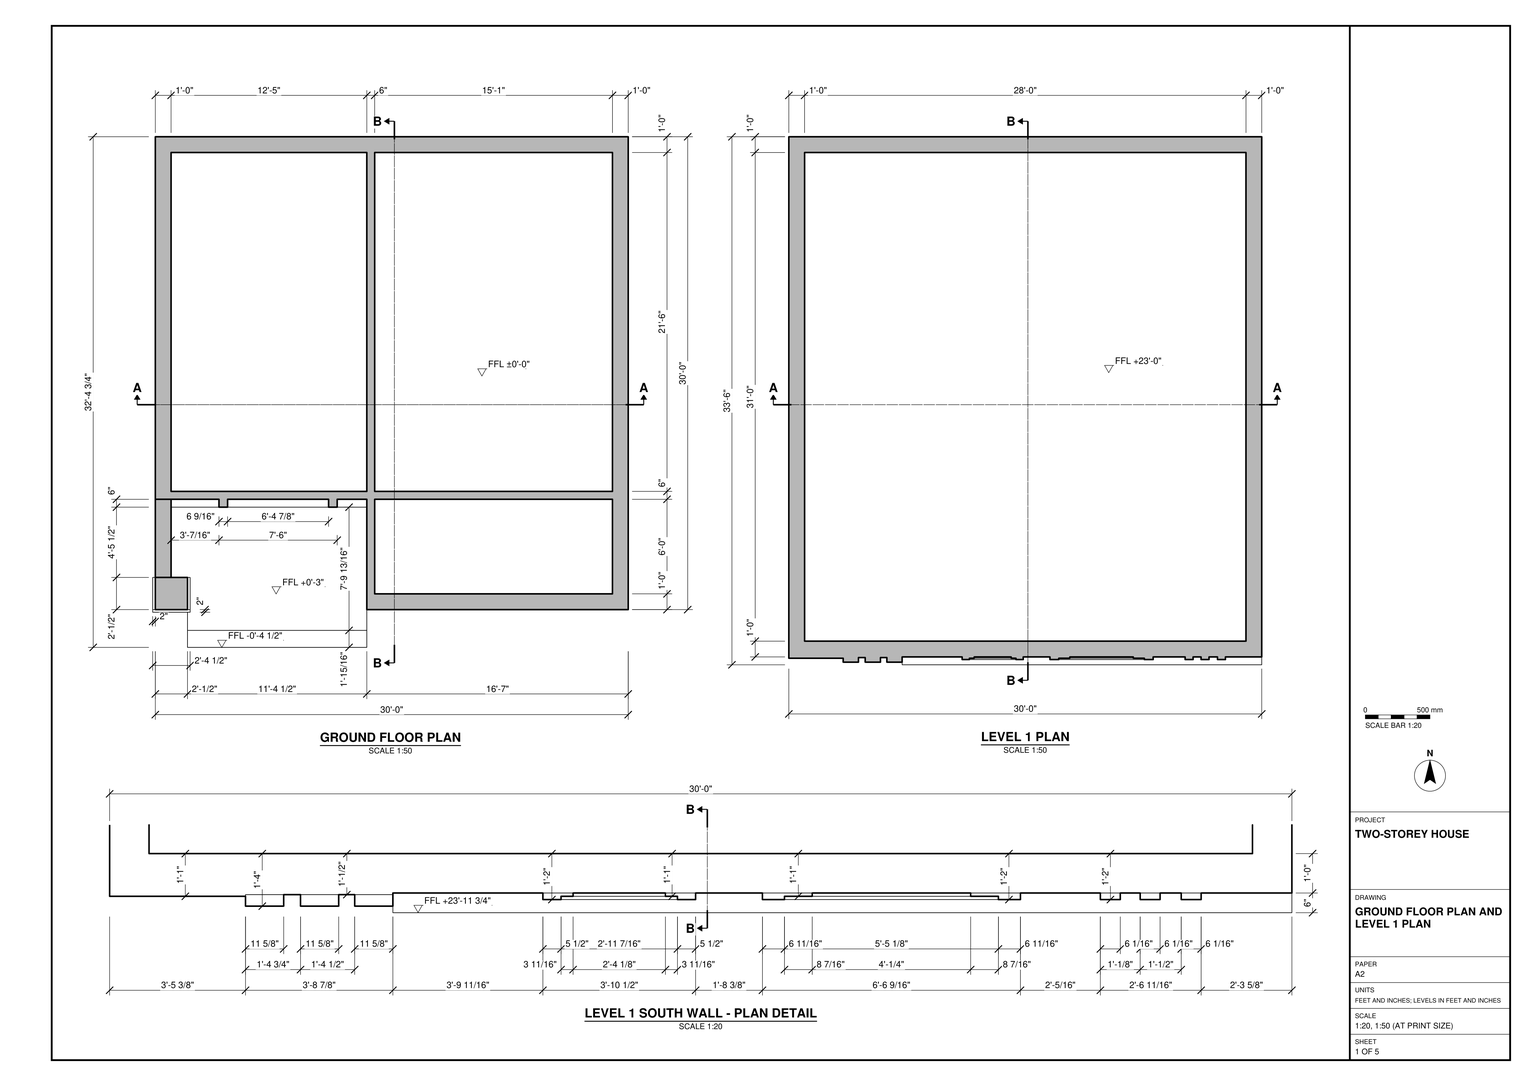
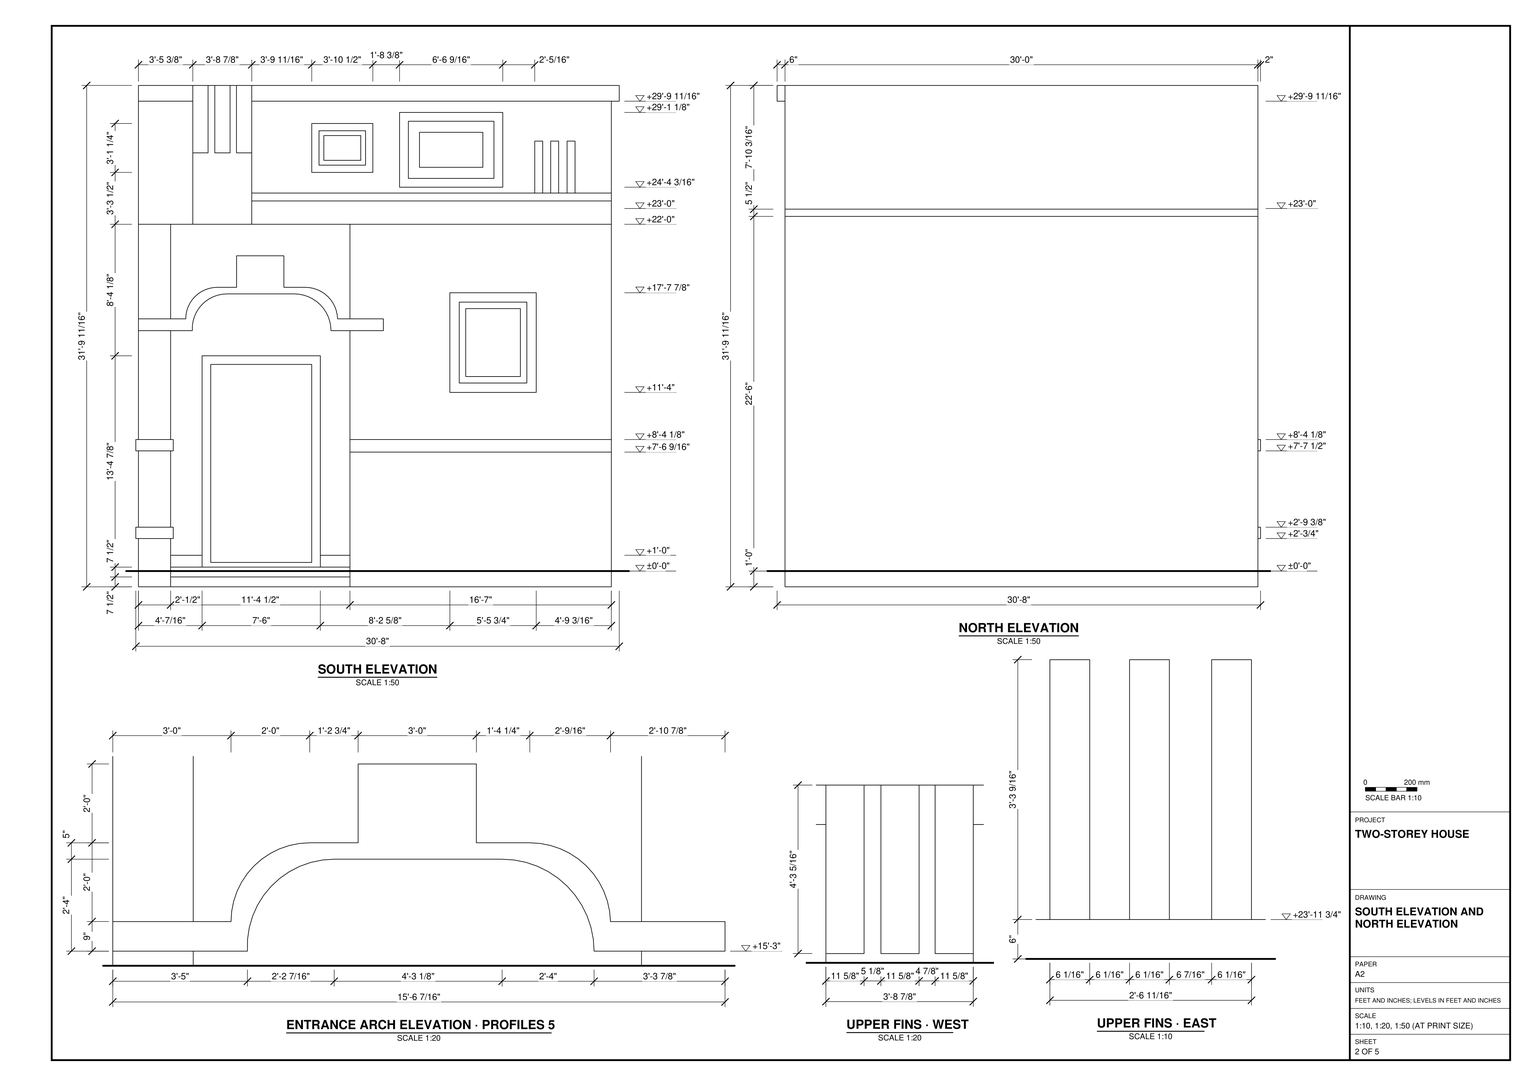
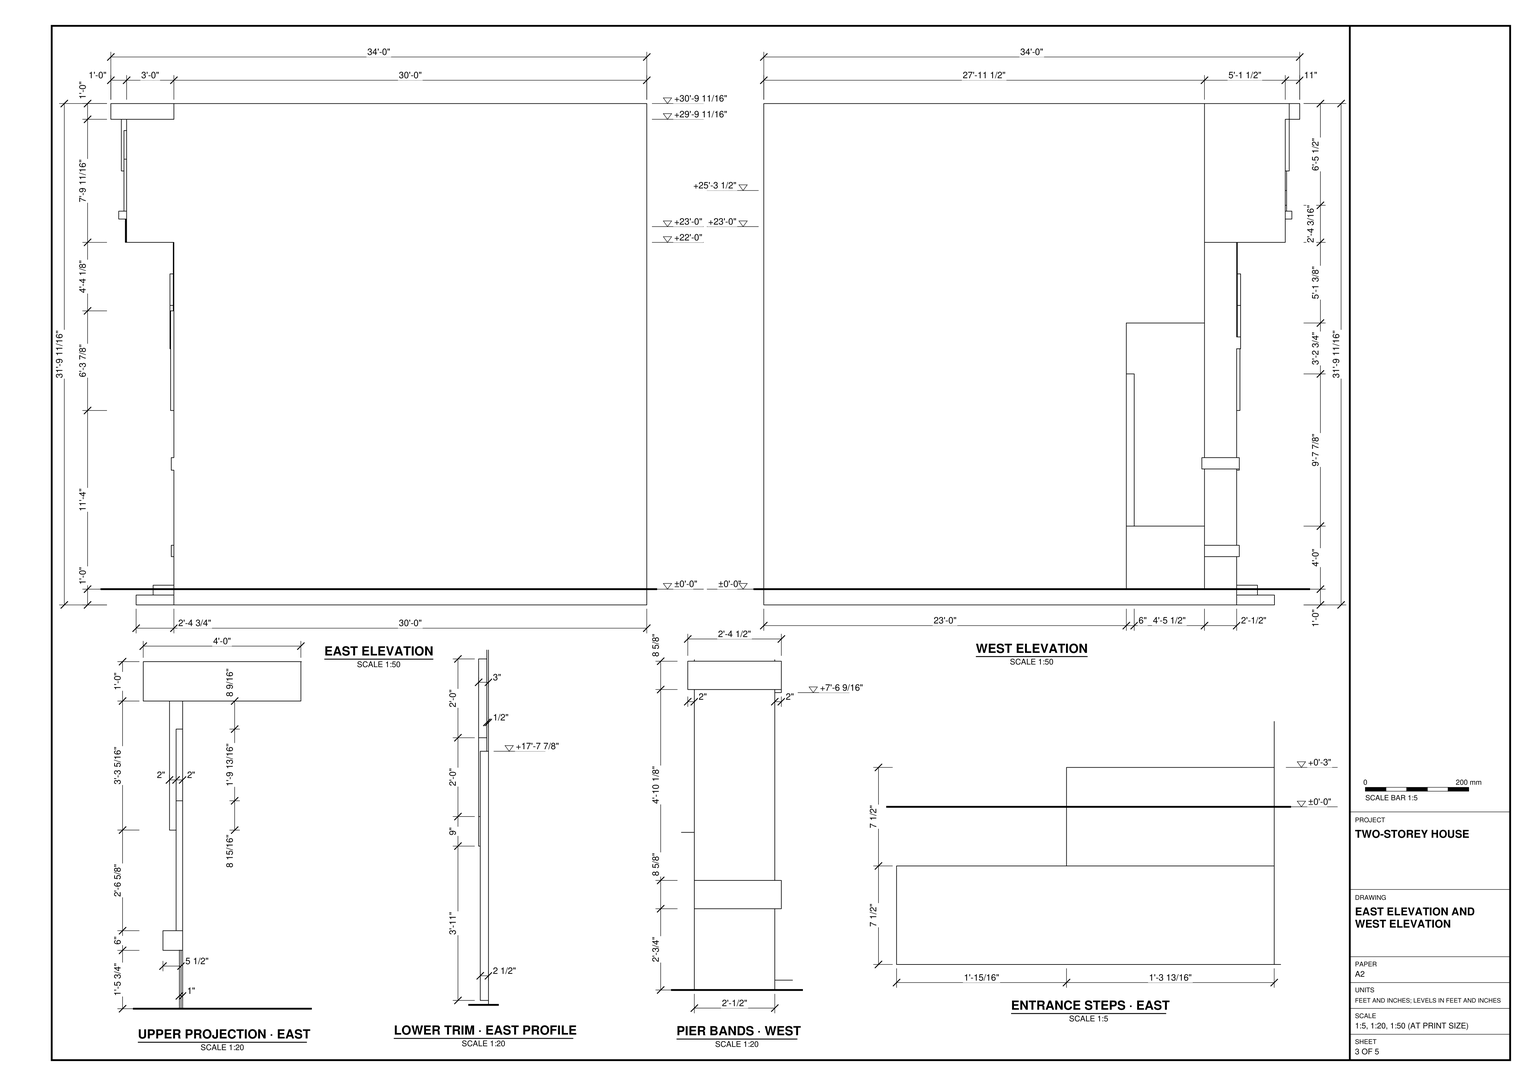
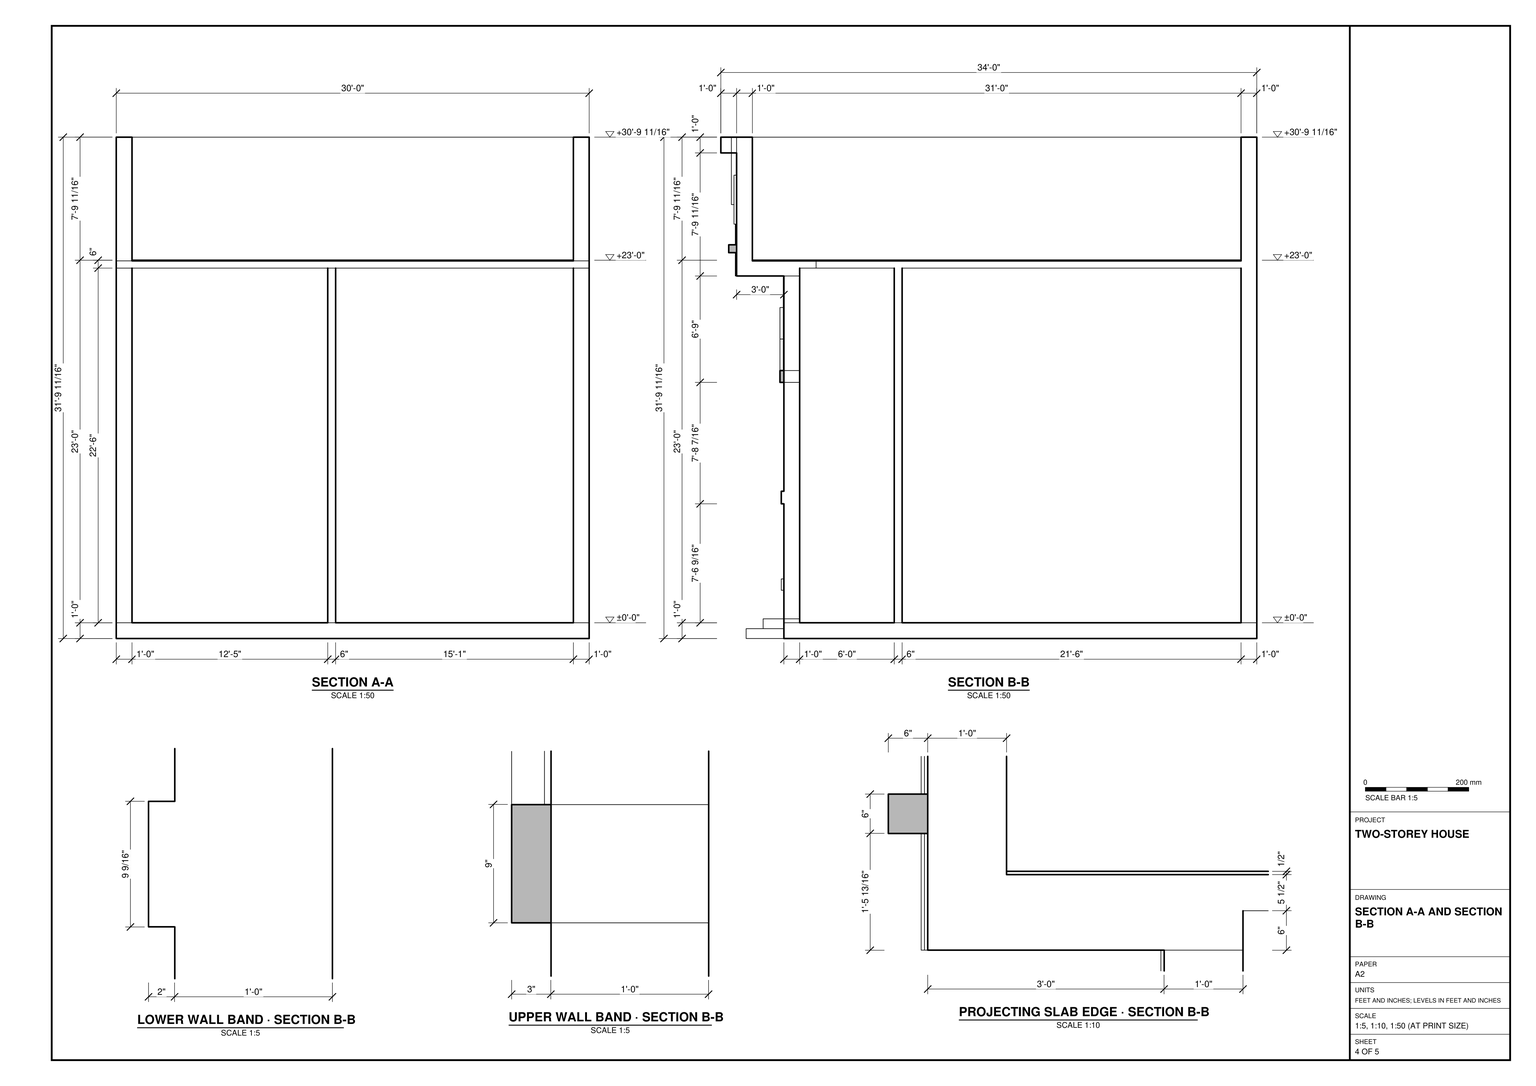
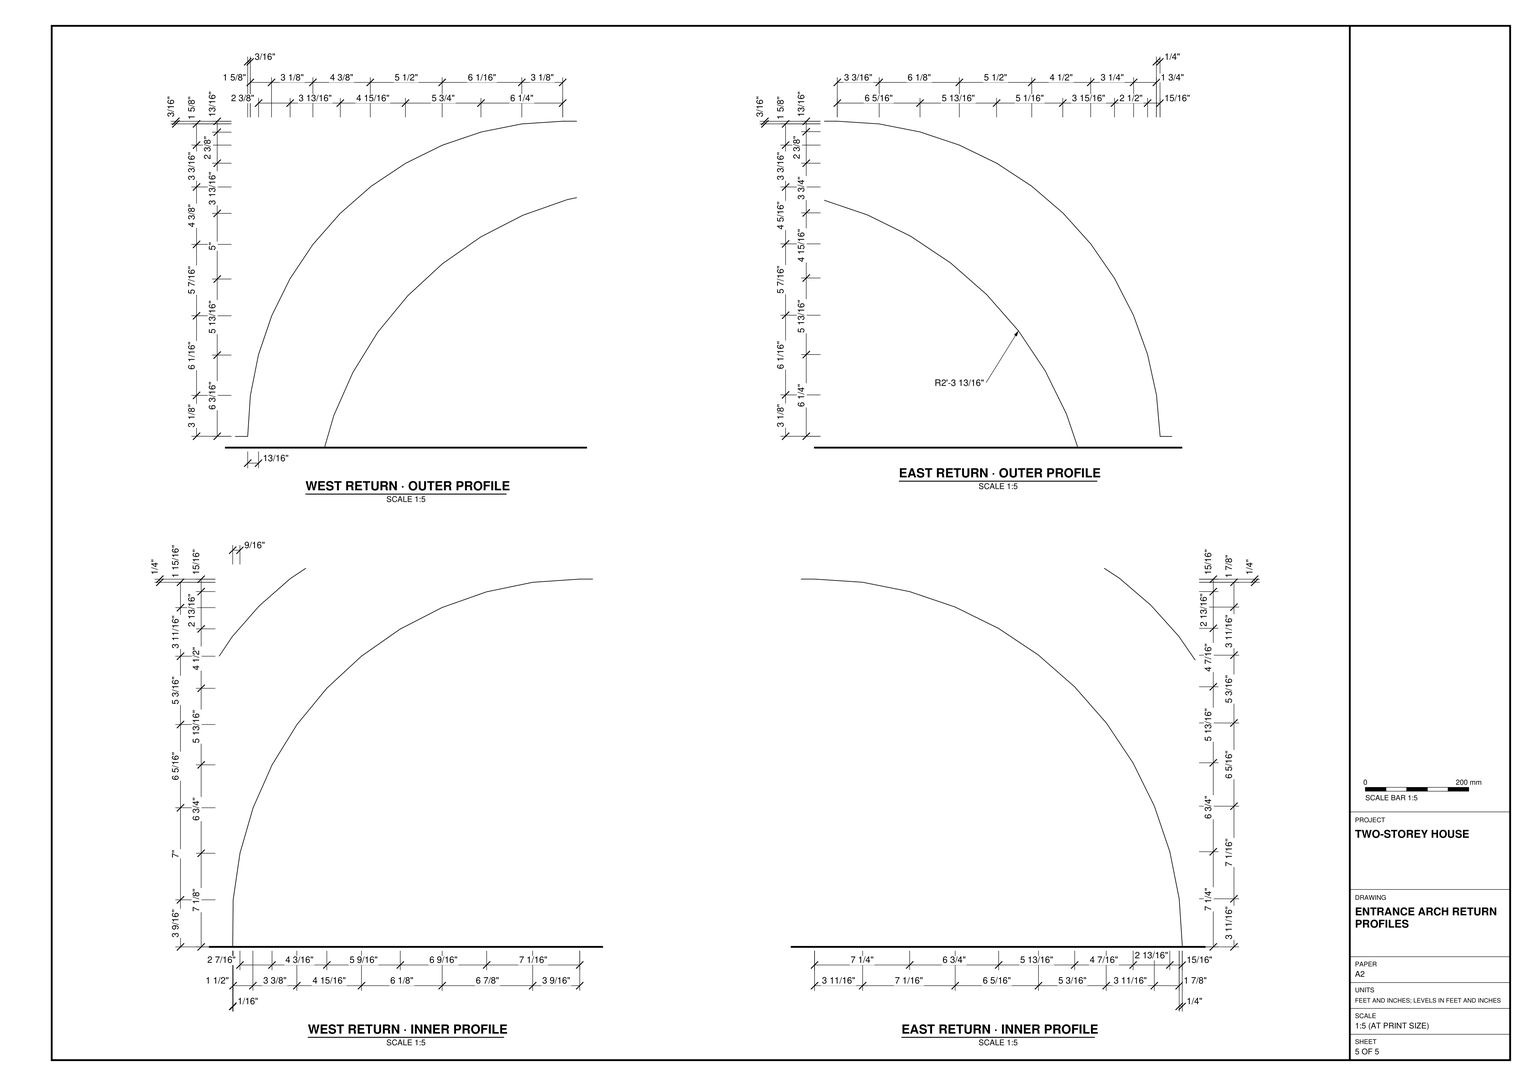
Build the two-storey house in SketchUp from task_files/diagram_01.pdf. Work in feet and inches. Including projections, the house measures 30'-8" east to west, 34'-0" north to south and 31'-9 11/16" from bottom to top. Set the ground-floor level at ±0'-0" and the upper-floor level at +23'-0".

Lay out the ground floor with 1'-0" perimeter walls and 6" partitions. Place the two deep rooms side by side to the north, the shallow room to the southeast and the recessed entrance to the southwest. Model the floor slabs and entrance steps. Above the entrance, follow the elevation detail for the curved arch, its central raised block and the bands around the outer pier.

Keep the upper floor undivided as drawn. Project its south wall beyond the lower wall and carry the flat roof cap past it. Use the south wall plan detail with the elevation to give the framed panels, ledges and vertical fins their distinct depths and positions.

Keep walls, slabs and roof elements separate as groups or components. Keep each furniture or joinery piece shown separate and use components for repeated parts. Any decor or loose items shown may be suitable library components. Save one SketchUp model as output_files/two_storey_house_with_a_recessed_south_entrance.skp.

# SketchUp Ruby script. Lengths in inches.
U = 1.inch
M = Sketchup.active_model
def pt(a) = Geom::Point3d.new(a.map { |v| v * U })
def face(e, loops, mat)
  f = e.add_face(loops[0].map { |a| pt(a) })
  loops[1..].each { |l| e.add_face(l.map { |a| pt(a) }).erase! }
  f.material = f.back_material = mat if mat
  f
end
# faces: each face lists its corners as indices into pts; further lists are holes
def faces(e, pts, list, mat = nil) = list.each { |f| face(e, (f[0].is_a?(Array) ? f : [f]).map { |l| l.map { |i| pts[i] } }, mat) }
# xy, xz, yz: faces in a plane at the given z, y or x. An outline is a flat list of corners, or four numbers for a rectangle; further outlines are holes
def ring(l) = l.size == 4 ? [[l[0], l[1]], [l[2], l[1]], [l[2], l[3]], [l[0], l[3]]] : l.each_slice(2).to_a
def flat(e, list, mat, &to3) = list.each { |f| face(e, (f[0].is_a?(Array) ? f : [f]).map { |l| ring(l).map { |u, v| to3.(u, v) } }, mat) }
def xy(e, z, list, mat = nil) = flat(e, list, mat) { |x, y| [x, y, z] }
def xz(e, y, list, mat = nil) = flat(e, list, mat) { |x, z| [x, y, z] }
def yz(e, x, list, mat = nil) = flat(e, list, mat) { |y, z| [x, y, z] }
def lines(e, pts, list) = list.each { |a, b| e.add_line(pt(pts[a]), pt(pts[b])) }
# prism: a flat outline (further loops are holes) pulled along v
def prism(e, loops, v, mat = nil)
  f = face(e, loops, mat); d = Geom::Vector3d.new(v.map { |x| x * U })
  f.pushpull(f.normal.samedirection?(d) ? d.length : -d.length)
end
def box(e, o, s, mat = nil) = prism(e, [[o, [o[0] + s[0], o[1], o[2]], [o[0] + s[0], o[1] + s[1], o[2]], [o[0], o[1] + s[1], o[2]]]], [0, 0, s[2]], mat)
def at(x, y, z, deg = 0) = Geom::Transformation.translation(pt([x, y, z])) * Geom::Transformation.rotation(ORIGIN, Z_AXIS, deg.degrees)
def axes(o, x, y, z) = Geom::Transformation.new([*x, 0, *y, 0, *z, 0, *pt(o).to_a, 1])
def part(name) = M.definitions.add(name)
# library, detail: a bought-in or finely detailed component or shape, given as its bounding box
def library(name, o, s) = part(name).tap { |d| box(d.entities, o, s) }
def detail(e, o, s) = box(e.add_group.entities, o, s)
def put(e, d, t, mat = nil) = e.add_instance(d, t).tap { |i| i.material = mat if mat }
def group(e, t, mat = nil) = e.add_group.tap { |g| g.transformation = t; g.material = mat if mat }.entities
root = M.entities
M.materials.add("[0004_HotPink]").color = [226, 93, 160]
M.materials.add("[0012_Bisque]").color = [211, 189, 162]
M.materials.add("[0017_IndianRed]").color = [99, 44, 44]
M.materials.add("[0111_SlateGray]").color = [112, 128, 144]
M.materials.add("[0118_Thistle]").color = [216, 191, 216]
M.materials.add("[0119_RosyBrown]").color = [188, 143, 143]
M.materials.add("[Carrera Marble]").color = [155, 155, 155]
M.materials.add("[Concrete Aggregate Smoke]").color = [154, 150, 148]
M.materials.add("[Crushed Rock Gravel]").color = [94, 94, 94]
M.materials.add("[Wood Cherry Original]").color = [152, 86, 42]
g1 = group(root,at(0,0,0))
xy(g1,0,[[26.5,19.25,26.5,48,2,48,2,408,362,408,362,48,163,48,163,19.25]])
xy(g1,7.5,[[26.5,19.25,163,32.1875]],"[Carrera Marble]")
xy(g1,12,[[169,60,350,132],[14,126,50.45,132],[140.45,126,163,132],[14,138,163,396],[169,138,350,396]])
xy(g1,15,[[26.5,32.1875,163,32.1875,163,126,14,126,14,72.5,26.5,72.5]],"[Carrera Marble]")
xy(g1,18.5625,[[57.02,126,133.89,132]],"[0017_IndianRed]")
xy(g1,24,[[140.45,126,163,132]])
xy(g1,24,[[14,126,50.45,132]],"[Carrera Marble]")
xy(g1,36.75,[[0,46,28.5,48],[0,48,2,72.5],[26.5,48,28.5,72.5]])
xy(g1,45.37,[[0,46,28.5,48],[0,48,2,72.5],[26.5,48,28.5,72.5]],"[0111_SlateGray]")
xy(g1,60,[[2,72.5,14,132]],"[0111_SlateGray]")
xy(g1,102.57,[[163,46,362,48]],"[Concrete Aggregate Smoke]")
xy(g1,103.5,[[0,46,28.5,48],[0,48,2,74.5],[2,48,26.5,72.5],[26.5,48,28.5,74.5],[2,72.5,26.5,74.5]])
xy(g1,112.12,[[0,48,2,74.5],[2,48,26.5,72.5],[2,72.5,26.5,74.5]])
xy(g1,112.12,[[0,46,28.5,48],[26.5,48,28.5,74.5]],"[0111_SlateGray]")
xy(g1,112.12,[[163,46,362,48]],"[Concrete Aggregate Smoke]")
xy(g1,148,[[239.06,45.5,304.81,48]],"[0017_IndianRed]")
xy(g1,155.14,[[246.2,45.5,297.67,46.5]])
xy(g1,160.07,[[251.13,46.5,292.73,48]],"[Concrete Aggregate Smoke]")
xy(g1,169.3125,[[57.02,126,133.89,132]],"[0017_IndianRed]")
xy(g1,175.875,[[50.45,126,140.45,132]],"[0017_IndianRed]")
xy(g1,195,[[2,45,2,48,26.5,48,26.5,60.25,43,60.25,43,45],[148.5625,45,148.5625,60.25,163,60.25,163,48,188.4375,48,188.4375,45]],"[0119_RosyBrown]")
xy(g1,204,[[26.5,47.5,38,48],[153.5625,47.5,163,48]])
xy(g1,204,[[2,45,38,45,38,47.5,26.5,47.5,26.5,48,2,48],[153.5625,45,163,47.5],[163,45,188.4375,48]],"[0119_RosyBrown]")
xy(g1,211.8,[[251.13,46.5,292.73,48]],"[Concrete Aggregate Smoke]")
xy(g1,214.61,[[2,72.5,14,132]])
xy(g1,216.74,[[246.2,45.5,297.67,46.5]])
xy(g1,223,[[69.42,45,120.5625,60.25]],"[0119_RosyBrown]")
xy(g1,223.875,[[239.06,45.5,304.81,48]],"[0017_IndianRed]")
xy(g1,228,[[62,47.5,76.71,48],[112.71,47.5,129,48]])
xy(g1,228,[[62,45,76.71,47.5],[112.71,45,129,47.5]],"[0119_RosyBrown]")
xy(g1,252,[[76.71,47.5,112.71,48]])
xy(g1,252,[[76.71,45,112.71,47.5]],"[0119_RosyBrown]")
xy(g1,276,[[26.5,47.5,163,48]])
xy(g1,276,[[2,11,2,48,26.5,48,26.5,47.5,163,47.5,163,48,362,48,362,12,88.25,12,88.25,11.5,43.375,11.5,43.375,11]],"[0118_Thistle]")
xy(g1,287.5,[[14,24,350,396]])
xy(g1,288,[[14,24,350,396]])
xy(g1,293.76,[[88.25,6,362,12]],"[Concrete Aggregate Smoke]")
xy(g1,299.76,[[303.68,10,309.74,12],[315.81,10,321.87,12],[328.31,10,334.37,12]])
xy(g1,299.76,[[88.25,6,362,6,362,12,334.37,12,334.37,10,328.31,10,328.31,12,321.87,12,321.87,10,315.81,10,315.81,12,309.74,12,309.74,10,303.68,10,303.68,12,88.25,12]],"[Concrete Aggregate Smoke]")
xy(g1,304.21,[[200.78,10,279.34,12]])
xy(g1,310.92,[[207.49,10,272.63,11]],"[0012_Bisque]")
xy(g1,315.48,[[133.93,10,180.43,12]])
xy(g1,319.37,[[215.93,11,264.1875,12]])
xy(g1,321.01,[[139.45,10,174.9,11]],"[0012_Bisque]")
xy(g1,324.67,[[143.12,11,171.24,12]])
xy(g1,330.375,[[43.375,8,55,11.5],[60.125,8,71.75,11.5],[76.625,8,88.25,11.5]],"[0012_Bisque]")
xy(g1,339.32,[[303.68,10,309.74,12],[315.81,10,321.87,12],[328.31,10,334.37,12]],"[0012_Bisque]")
xy(g1,343.54,[[143.12,11,171.24,12]])
xy(g1,346,[[215.93,11,264.1875,12]])
xy(g1,347.21,[[139.45,10,174.9,11]],"[0012_Bisque]")
xy(g1,352.73,[[133.93,10,180.43,12]],"[0012_Bisque]")
xy(g1,354.44,[[207.49,10,272.63,11]],"[0012_Bisque]")
xy(g1,361.15,[[200.78,10,279.34,12]],"[0012_Bisque]")
xy(g1,369.6875,[[2,8,43.375,11],[362,12,368,48]])
xy(g1,369.6875,[[88.25,0,362,12],[362,0,368,12]],"[0118_Thistle]")
xy(g1,381.6875,[[[88.25,0,368,0,368,48,362,48,362,408,2,408,2,8,55,8,55,11.5,60.125,11.5,60.125,8,71.75,8,71.75,11.5,76.625,11.5,76.625,8,87.75,8,87.75,12,88.25,12],[14,24,350,396]],[87.75,8,88.25,12]])
xz(g1,0,[[88.25,369.6875,368,381.6875]],"[0118_Thistle]")
xz(g1,6,[[88.25,293.76,362,299.76]],"[Concrete Aggregate Smoke]")
xz(g1,8,[[2,369.6875,43.375,381.6875]],"[0004_HotPink]")
xz(g1,8,[[43.375,330.375,55,381.6875],[60.125,330.375,71.75,381.6875],[76.625,330.375,88.25,381.6875]],"[0012_Bisque]")
xz(g1,10,[[303.68,299.76,309.74,339.32],[315.81,299.76,321.87,339.32],[328.31,299.76,334.37,339.32],[[200.78,304.21,279.34,361.15],[207.49,310.92,272.63,354.44]],[[133.93,315.48,180.43,352.73],[139.45,321.01,174.9,347.21]]],"[0012_Bisque]")
xz(g1,11,[[2,276,43.375,369.6875]],"[0118_Thistle]")
xz(g1,11,[[[207.49,310.92,272.63,354.44],[215.93,319.37,264.1875,346]],[[139.45,321.01,174.9,347.21],[143.12,324.67,171.24,343.54]]],"[0119_RosyBrown]")
xz(g1,11.5,[[43.375,276,88.25,276,88.25,330.375,76.625,330.375,76.625,381.6875,71.75,381.6875,71.75,330.375,60.125,330.375,60.125,381.6875,55,381.6875,55,330.375,43.375,330.375]],"[0004_HotPink]")
xz(g1,12,[[88.25,293.76,362,299.76],[87.75,369.6875,88.25,381.6875]])
xz(g1,12,[[88.25,276,362,293.76],[[88.25,299.76,303.68,299.76,303.68,339.32,309.74,339.32,309.74,299.76,315.81,299.76,315.81,339.32,321.87,339.32,321.87,299.76,328.31,299.76,328.31,339.32,334.37,339.32,334.37,299.76,362,299.76,362,369.6875,88.25,369.6875],[200.78,304.21,279.34,361.15],[133.93,315.48,180.43,352.73]]],"[0118_Thistle]")
xz(g1,12,[[215.93,319.37,264.1875,346],[143.12,324.67,171.24,343.54]],"[Concrete Aggregate Smoke]")
xz(g1,19.25,[[26.5,0,163,7.5]],"[Carrera Marble]")
xz(g1,24,[[14,287.5,350,288],[14,288,350,381.6875]])
xz(g1,32.1875,[[26.5,7.5,163,15]],"[Carrera Marble]")
xz(g1,45,[[2,195,43,195,43.04,198.59,43.56,202.14,44.09,204,44.55,205.59,46.01,208.87,47.89,211.93,50.17,214.7,52.81,217.14,55.75,219.19,58.9375,220.84,62.32,222.03,65.84,222.76,69.42,223,120.5625,223,124.22,222.76,127.81,222.05,131.28,220.87,134.5625,219.25,137.61,217.21,140.36,214.8,142.78,212.05,144.8125,209,146.43,205.72,147.01,204,147.61,202.25,148.32,198.65,148.5625,195,188.4375,195,188.4375,204,153.5625,204,153.29,207.15,152.61,210.25,151.53,213.23,150.09,216.04,148.5625,218.25,148.29,218.65,146.17,221,143.85,223,143.77,223.07,141.12,224.8,138.27,226.18,135.27,227.1875,132.16,227.8,129,228,112.71,228,112.71,252,76.71,252,76.71,228,62,228,58.87,227.79,55.79,227.18,52.82,226.17,50,224.78,47.39,223.04,47.34,223,45.03,220.97,43,218.66,42.96,218.61,41.22,216,39.83,213.18,38.82,210.21,38.21,207.13,38,204,2,204]],"[0119_RosyBrown]")
xz(g1,45.5,[[[239.06,148,304.81,223.875],[246.2,155.14,297.67,216.74]]],"[0017_IndianRed]")
xz(g1,46,[[0,36.75,28.5,45.37],[0,103.5,28.5,112.12]],"[0111_SlateGray]")
xz(g1,46,[[163,102.57,362,112.12]],"[Concrete Aggregate Smoke]")
xz(g1,46.5,[[[246.2,155.14,297.67,216.74],[251.13,160.07,292.73,211.8]]],"[0119_RosyBrown]")
xz(g1,47.5,[[26.5,204,38,204,38.21,207.13,38.82,210.21,39.83,213.18,41.22,216,42.96,218.61,43,218.66,45.03,220.97,47.34,223,47.39,223.04,50,224.78,52.82,226.17,55.79,227.18,58.87,227.79,62,228,76.71,228,76.71,252,112.71,252,112.71,228,129,228,132.16,227.8,135.27,227.1875,138.27,226.18,141.12,224.8,143.77,223.07,143.85,223,146.17,221,148.29,218.65,148.5625,218.25,150.09,216.04,151.53,213.23,152.61,210.25,153.29,207.15,153.5625,204,163,204,163,276,26.5,276]],"[0118_Thistle]")
xz(g1,48,[[163,195,188.4375,204],[26.5,204,38,204,38.21,207.13,38.82,210.21,39.83,213.18,41.22,216,42.96,218.61,43,218.66,45.03,220.97,47.34,223,47.39,223.04,50,224.78,52.82,226.17,55.79,227.18,58.87,227.79,62,228,76.71,228,76.71,252,112.71,252,112.71,228,129,228,132.16,227.8,135.27,227.1875,138.27,226.18,141.12,224.8,143.77,223.07,143.85,223,146.17,221,148.29,218.65,148.5625,218.25,150.09,216.04,151.53,213.23,152.61,210.25,153.29,207.15,153.5625,204,163,204,163,276,26.5,276],[362,369.6875,368,381.6875]])
xz(g1,48,[[163,0,362,102.57],[[163,112.12,362,112.12,362,276,163,276,163,204,188.4375,204,188.4375,195,163,195],[239.06,148,304.81,223.875]]],"[0118_Thistle]")
xz(g1,48,[[251.13,160.07,292.73,211.8]],"[Concrete Aggregate Smoke]")
xz(g1,48,[[2,0,26.5,36.75],[2,45.37,26.5,103.5],[2,112.12,26.5,195],[2,204,26.5,276]],"[Crushed Rock Gravel]")
xz(g1,60,[[169,12,350,282]])
xz(g1,60.25,[[26.5,195,26.5,282,163,282,163,195,148.5625,195,148.32,198.65,147.61,202.25,147.01,204,146.43,205.72,144.8125,209,142.78,212.05,140.36,214.8,137.61,217.21,134.5625,219.25,131.28,220.87,127.81,222.05,124.22,222.76,120.5625,223,69.42,223,65.84,222.76,62.32,222.03,58.9375,220.84,55.75,219.19,52.81,217.14,50.17,214.7,47.89,211.93,46.01,208.87,44.55,205.59,44.09,204,43.56,202.14,43.04,198.59,43,195]])
xz(g1,72.5,[[2,12,14,36.75],[14,15,26.5,36.75],[0,36.75,2,45.37],[2,36.75,14,45.37],[14,36.75,28.5,45.37],
  [2,45.37,14,60]])
xz(g1,72.5,[[14,45.37,14,60,2,60,2,103.5,26.5,103.5,26.5,45.37],[2,112.12,2,214.61,14,214.61,14,282,26.5,282,26.5,112.12]],"[Crushed Rock Gravel]")
xz(g1,74.5,[[0,103.5,28.5,112.12]])
xz(g1,126,[[14,12,50.45,15],[140.45,12,163,15]])
xz(g1,126,[[[50.45,15,140.45,175.875],[57.02,18.5625,133.89,169.3125]]],"[0017_IndianRed]")
xz(g1,126,[[14,15,50.45,24],[140.45,15,163,24]],"[Carrera Marble]")
xz(g1,132,[[2,12,14,60],[14,12,50.45,24],[140.45,12,163,24],[169,12,350,282]])
xz(g1,132,[[14,24,50.45,24,50.45,175.875,140.45,175.875,140.45,24,163,24,163,282,14,282,14,214.61,2,214.61,2,60,14,60]],"[0118_Thistle]")
xz(g1,132,[[57.02,18.5625,133.89,169.3125]],"[Wood Cherry Original]")
xz(g1,138,[[14,12,163,282],[169,12,350,282]])
xz(g1,396,[[14,12,163,282],[169,12,350,282],[14,287.5,350,288],[14,288,350,381.6875]])
xz(g1,408,[[2,0,362,12],[2,12,362,282],[2,282,362,287.5],[2,287.5,362,381.6875]])
yz(g1,0,[[46,103.5,74.5,112.12]])
yz(g1,0,[[46,36.75,72.5,45.37]],"[0111_SlateGray]")
yz(g1,2,[[132,12,132,214.61,72.5,214.61,72.5,381.6875,408,381.6875,408,12],[11,276,11,369.6875,8,369.6875,8,381.6875,72.5,381.6875,72.5,276]])
yz(g1,2,[[48,0,48,12,72.5,12,72.5,60,132,60,132,12,408,12,408,0],[48,12,72.5,36.75]],"[0111_SlateGray]")
yz(g1,2,[[48,45.37,72.5,103.5],[48,112.12,48,195,45,195,45,204,48,204,48,276,72.5,276,72.5,112.12]],"[Crushed Rock Gravel]")
yz(g1,14,[[138,12,396,282],[72.5,15,126,15,126,24,132,24,132,60,72.5,60],[72.5,214.61,132,282],[24,287.5,396,288],[24,288,396,381.6875]])
yz(g1,26.5,[[19.25,0,48,7.5],[32.1875,7.5,48,15],[48,195,60.25,204],[47.5,204,48,276],[48,204,60.25,276]])
yz(g1,26.5,[[48,15,72.5,36.75],[48,45.37,72.5,103.5],[48,112.12,72.5,112.12,72.5,282,60.25,282,60.25,195,48,195]],"[Crushed Rock Gravel]")
yz(g1,28.5,[[46,36.75,72.5,45.37],[46,103.5,74.5,112.12]],"[0111_SlateGray]")
yz(g1,43.375,[[11,276,11.5,330.375]])
yz(g1,43.375,[[8,330.375,11,369.6875]],"[0012_Bisque]")
yz(g1,50.45,[[126,12,132,24]])
yz(g1,50.45,[[126,24,132,175.875]],"[0017_IndianRed]")
yz(g1,55,[[8,330.375,11.5,381.6875]],"[0012_Bisque]")
yz(g1,57.02,[[126,18.5625,132,169.3125]],"[0017_IndianRed]")
yz(g1,60.125,[[8,330.375,11.5,381.6875]],"[0012_Bisque]")
yz(g1,71.75,[[8,330.375,11.5,381.6875]],"[0012_Bisque]")
yz(g1,76.625,[[8,330.375,11.5,381.6875]],"[0012_Bisque]")
yz(g1,76.71,[[47.5,228,48,252]])
yz(g1,76.71,[[45,228,47.5,252]],"[0119_RosyBrown]")
yz(g1,88.25,[[11.5,276,12,293.76],[11.5,293.76,12,299.76],[11.5,299.76,12,330.375],[8,369.6875,12,381.6875]])
yz(g1,88.25,[[8,330.375,12,369.6875]],"[0012_Bisque]")
yz(g1,88.25,[[6,293.76,11.5,299.76],[0,369.6875,8,381.6875]],"[0118_Thistle]")
yz(g1,112.71,[[47.5,228,48,252]])
yz(g1,112.71,[[45,228,47.5,252]],"[0119_RosyBrown]")
yz(g1,133.89,[[126,18.5625,132,169.3125]],"[0017_IndianRed]")
yz(g1,133.93,[[10,315.48,12,352.73]],"[0012_Bisque]")
yz(g1,139.45,[[10,321.01,11,347.21]],"[0012_Bisque]")
yz(g1,140.45,[[126,12,132,24]])
yz(g1,140.45,[[126,24,132,175.875]],"[0017_IndianRed]")
yz(g1,143.12,[[11,324.67,12,343.54]])
yz(g1,163,[[19.25,0,48,7.5],[32.1875,7.5,48,15],[138,12,396,282],[48,195,60.25,204],[47.5,204,48,276],
  [48,204,60.25,276]])
yz(g1,163,[[48,15,48,102.57,46,102.57,46,112.12,48,112.12,48,195,60.25,195,60.25,282,132,282,132,24,126,24,126,15]],"[0118_Thistle]")
yz(g1,169,[[60,12,132,282],[138,12,396,282]])
yz(g1,171.24,[[11,324.67,12,343.54]])
yz(g1,174.9,[[10,321.01,11,347.21]],"[0012_Bisque]")
yz(g1,180.43,[[10,315.48,12,352.73]],"[0012_Bisque]")
yz(g1,188.4375,[[45,195,48,204]],"[0119_RosyBrown]")
yz(g1,200.78,[[10,304.21,12,361.15]],"[0012_Bisque]")
yz(g1,207.49,[[10,310.92,11,354.44]],"[0012_Bisque]")
yz(g1,215.93,[[11,319.37,12,346]])
yz(g1,239.06,[[45.5,148,48,223.875]],"[0017_IndianRed]")
yz(g1,246.2,[[45.5,155.14,46.5,216.74]],"[0017_IndianRed]")
yz(g1,251.13,[[46.5,160.07,48,211.8]],"[Concrete Aggregate Smoke]")
yz(g1,264.1875,[[11,319.37,12,346]])
yz(g1,272.63,[[10,310.92,11,354.44]],"[0012_Bisque]")
yz(g1,279.34,[[10,304.21,12,361.15]],"[0012_Bisque]")
yz(g1,292.73,[[46.5,160.07,48,211.8]],"[Concrete Aggregate Smoke]")
yz(g1,297.67,[[45.5,155.14,46.5,216.74]])
yz(g1,303.68,[[10,299.76,12,339.32]],"[0012_Bisque]")
yz(g1,304.81,[[45.5,148,48,223.875]],"[0017_IndianRed]")
yz(g1,309.74,[[10,299.76,12,339.32]],"[0012_Bisque]")
yz(g1,315.81,[[10,299.76,12,339.32]],"[0012_Bisque]")
yz(g1,321.87,[[10,299.76,12,339.32]],"[0012_Bisque]")
yz(g1,328.31,[[10,299.76,12,339.32]],"[0012_Bisque]")
yz(g1,334.37,[[10,299.76,12,339.32]],"[0012_Bisque]")
yz(g1,350,[[60,12,132,282],[138,12,396,282],[24,287.5,396,288],[24,288,396,381.6875]])
yz(g1,362,[[48,0,408,12],[48,12,408,12,408,381.6875,48,381.6875,48,369.6875,12,369.6875,12,276,48,276,48,112.12,46,112.12,46,102.57,48,102.57],[6,293.76,12,299.76]])
yz(g1,368,[[0,369.6875,48,381.6875]])
p = [[43,45,195],[43,60.25,195],[43.04,60.25,198.59],[43.04,45,198.59],[148.32,45,198.65],[148.32,60.25,198.65],
  [148.5625,60.25,195],[148.5625,45,195],[43.56,60.25,202.14],[43.56,45,202.14],[147.61,45,202.25],[147.61,60.25,202.25],
  [44.09,60.25,204],[44.09,45,204],[147.01,45,204],[147.01,60.25,204],[38.21,45,207.13],[38.21,47.5,207.13],
  [38,47.5,204],[38,45,204],[44.55,60.25,205.59],[44.55,45,205.59],[146.43,45,205.72],[146.43,60.25,205.72],
  [153.5625,45,204],[153.5625,47.5,204],[153.29,47.5,207.15],[153.29,45,207.15],[38.21,48,207.13],[38,48,204],
  [153.5625,48,204],[153.29,48,207.15],[46.01,60.25,208.87],[46.01,45,208.87],[144.8125,45,209],[144.8125,60.25,209],
  [38.82,45,210.21],[38.82,47.5,210.21],[38.82,48,210.21],[152.61,47.5,210.25],[152.61,45,210.25],[152.61,48,210.25],
  [47.89,60.25,211.93],[47.89,45,211.93],[142.78,45,212.05],[142.78,60.25,212.05],[39.83,45,213.18],[39.83,47.5,213.18],
  [151.53,47.5,213.23],[151.53,45,213.23],[39.83,48,213.18],[151.53,48,213.23],[50.17,60.25,214.7],[50.17,45,214.7],
  [140.36,45,214.8],[140.36,60.25,214.8],[41.22,45,216],[41.22,47.5,216],[150.09,47.5,216.04],[150.09,45,216.04],
  [41.22,48,216],[150.09,48,216.04],[52.81,60.25,217.14],[52.81,45,217.14],[137.61,45,217.21],[137.61,60.25,217.21],
  [42.96,45,218.61],[42.96,47.5,218.61],[148.5625,47.5,218.25],[148.5625,45,218.25],[42.96,48,218.61],[148.5625,48,218.25],
  [55.75,60.25,219.19],[55.75,45,219.19],[134.5625,45,219.25],[134.5625,60.25,219.25],[148.29,47.5,218.65],[148.29,45,218.65],
  [148.29,48,218.65],[43,45,218.66],[43,47.5,218.66],[146.17,47.5,221],[146.17,45,221],[43,48,218.66],
  [146.17,48,221],[45.03,45,220.97],[45.03,47.5,220.97],[45.03,48,220.97],[58.9375,60.25,220.84],[58.9375,45,220.84],
  [131.28,45,220.87],[131.28,60.25,220.87],[62.32,60.25,222.03],[62.32,45,222.03],[127.81,45,222.05],[127.81,60.25,222.05],
  [47.34,45,223],[47.34,47.5,223],[143.85,47.5,223],[143.85,45,223],[47.34,48,223],[143.85,48,223],
  [65.84,60.25,222.76],[65.84,45,222.76],[124.22,45,222.76],[124.22,60.25,222.76],[69.42,60.25,223],[69.42,45,223],
  [120.5625,45,223],[120.5625,60.25,223],[47.39,45,223.04],[47.39,47.5,223.04],[50,45,224.78],[50,47.5,224.78],
  [143.77,47.5,223.07],[143.77,45,223.07],[47.39,48,223.04],[50,48,224.78],[143.77,48,223.07],[141.12,47.5,224.8],
  [141.12,45,224.8],[141.12,48,224.8],[52.82,45,226.17],[52.82,47.5,226.17],[138.27,47.5,226.18],[138.27,45,226.18],
  [52.82,48,226.17],[138.27,48,226.18],[55.79,45,227.18],[55.79,47.5,227.18],[135.27,47.5,227.1875],[135.27,45,227.1875],
  [55.79,48,227.18],[135.27,48,227.1875],[58.87,45,227.79],[58.87,47.5,227.79],[132.16,47.5,227.8],[132.16,45,227.8],
  [58.87,48,227.79],[132.16,48,227.8],[62,45,228],[62,47.5,228],[129,47.5,228],[129,45,228],
  [62,48,228],[129,48,228],[112.71,48,228],[112.71,60.25,228],[38,60.25,204],[76.71,48,252],
  [76.71,60.25,252],[62,60.25,228],[112.71,48,252],[112.71,60.25,252],[169,48,276],[169,60,276],
  [169,48,12],[169,60,12],[14,132,282],[2,132,282],[362,12,369.6875],[362,12,381.6875],
  [163,396,282],[169,396,282],[87.75,8,369.6875],[87.75,12,369.6875],[350,138,282],[350,132,282]]
faces(g1,p,[[0,1,2,3],[4,5,6,7],[3,2,8,9],[10,11,5,4],[9,8,12,13],[14,15,11,10],[16,17,18,19],[13,12,20,21],
  [22,23,15,14],[24,25,26,27],[21,20,32,33],[34,35,23,22],[36,37,17,16],[27,26,39,40],[33,32,42,43],[44,45,35,34],
  [46,47,37,36],[40,39,48,49],[43,42,52,53],[54,55,45,44],[56,57,47,46],[49,48,58,59],[53,52,62,63],[64,65,55,54],
  [66,67,57,56],[59,58,68,69],[63,62,72,73],[74,75,65,64],[69,68,76,77],[79,80,67,66],[77,76,81,82],[85,86,80,79],
  [73,72,88,89],[90,91,75,74],[89,88,92,93],[94,95,91,90],[96,97,86,85],[82,81,98,99],[93,92,102,103],[104,105,95,94],
  [103,102,106,107],[108,109,105,104],[110,111,97,96],[112,113,111,110],[99,98,114,115],[115,114,119,120],[122,123,113,112],[120,119,124,125],
  [128,129,123,122],[125,124,130,131],[134,135,129,128],[131,130,136,137],[140,141,135,134],[137,136,142,143]],"[0119_RosyBrown]")
faces(g1,p,[[28,29,18,17],[30,31,26,25],[38,28,17,37],[31,41,39,26],[50,38,37,47],[41,51,48,39],[60,50,47,57],[51,61,58,48],
  [70,60,57,67],[61,71,68,58],[71,78,76,68],[83,70,67,80],[78,84,81,76],[87,83,80,86],[100,87,86,97],[84,101,98,81],
  [116,100,97,111],[117,116,111,113],[101,118,114,98],[118,121,119,114],[126,117,113,123],[121,127,124,119],[132,126,123,129],[127,133,130,124],
  [138,132,129,135],[133,139,136,130],[144,138,135,141],[139,145,142,136]])
lines(g1,p,[[146,147],[29,148],[149,150],[144,151],[152,153],[154,155],[156,157],[158,159],[160,161],[162,163],[164,165],[166,167]])
